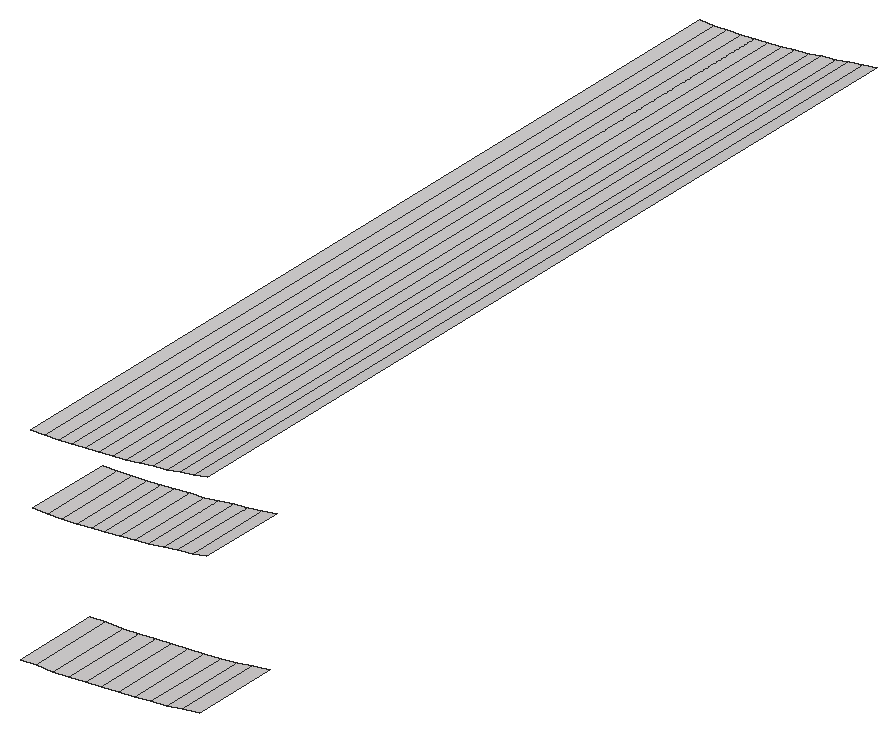
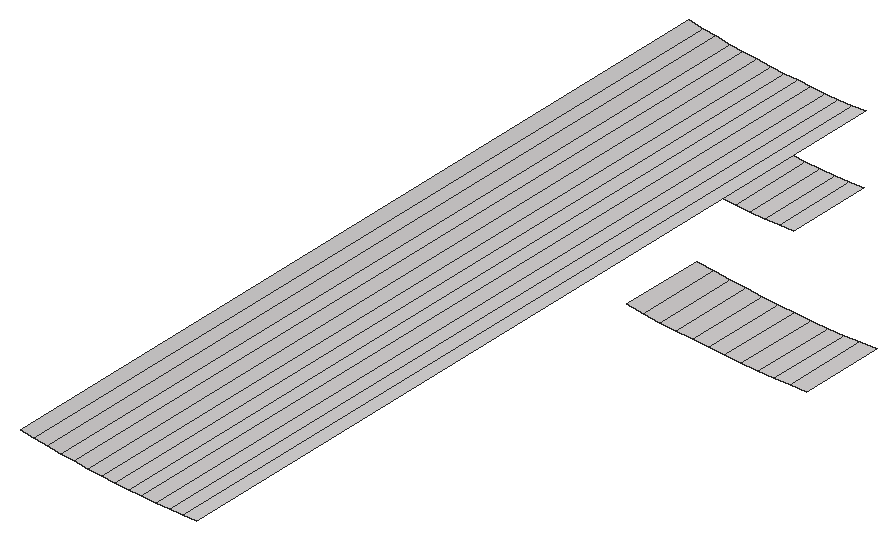
# SketchUp Ruby script. Lengths in inches.
U = 1.inch
M = Sketchup.active_model
def pt(a) = Geom::Point3d.new(a.map { |v| v * U })
def face(e, loops, mat)
  f = e.add_face(loops[0].map { |a| pt(a) })
  loops[1..].each { |l| e.add_face(l.map { |a| pt(a) }).erase! }
  f.material = f.back_material = mat if mat
  f
end
# faces: each face lists its corners as indices into pts; further lists are holes
def faces(e, pts, list, mat = nil) = list.each { |f| face(e, (f[0].is_a?(Array) ? f : [f]).map { |l| l.map { |i| pts[i] } }, mat) }
# xy, xz, yz: faces in a plane at the given z, y or x. An outline is a flat list of corners, or four numbers for a rectangle; further outlines are holes
def ring(l) = l.size == 4 ? [[l[0], l[1]], [l[2], l[1]], [l[2], l[3]], [l[0], l[3]]] : l.each_slice(2).to_a
def flat(e, list, mat, &to3) = list.each { |f| face(e, (f[0].is_a?(Array) ? f : [f]).map { |l| ring(l).map { |u, v| to3.(u, v) } }, mat) }
def xy(e, z, list, mat = nil) = flat(e, list, mat) { |x, y| [x, y, z] }
def xz(e, y, list, mat = nil) = flat(e, list, mat) { |x, z| [x, y, z] }
def yz(e, x, list, mat = nil) = flat(e, list, mat) { |y, z| [x, y, z] }
def lines(e, pts, list) = list.each { |a, b| e.add_line(pt(pts[a]), pt(pts[b])) }
# prism: a flat outline (further loops are holes) pulled along v
def prism(e, loops, v, mat = nil)
  f = face(e, loops, mat); d = Geom::Vector3d.new(v.map { |x| x * U })
  f.pushpull(f.normal.samedirection?(d) ? d.length : -d.length)
end
def box(e, o, s, mat = nil) = prism(e, [[o, [o[0] + s[0], o[1], o[2]], [o[0] + s[0], o[1] + s[1], o[2]], [o[0], o[1] + s[1], o[2]]]], [0, 0, s[2]], mat)
def at(x, y, z, deg = 0) = Geom::Transformation.translation(pt([x, y, z])) * Geom::Transformation.rotation(ORIGIN, Z_AXIS, deg.degrees)
def axes(o, x, y, z) = Geom::Transformation.new([*x, 0, *y, 0, *z, 0, *pt(o).to_a, 1])
def part(name) = M.definitions.add(name)
# library, detail: a bought-in or finely detailed component or shape, given as its bounding box
def library(name, o, s) = part(name).tap { |d| box(d.entities, o, s) }
def detail(e, o, s) = box(e.add_group.entities, o, s)
def put(e, d, t, mat = nil) = e.add_instance(d, t).tap { |i| i.material = mat if mat }
def group(e, t, mat = nil) = e.add_group.tap { |g| g.transformation = t; g.material = mat if mat }.entities
root = M.entities
M.materials.add("[Quartz Light Brown]").color = [215, 212, 212]
xy(root,150.01,[[450.47,143,450.71,144.25]],"[Quartz Light Brown]")
xy(root,152.01,[[450.42,143,450.63,144.25]],"[Quartz Light Brown]")
xy(root,153.01,[[450.39,143,450.59,155]],"[Quartz Light Brown]")
p = [[450.24,144.25,150],[450.24,143,150],[450.47,143,150.01],[450.47,144.25,150.01],[450.71,144.25,150.01],[450.71,143,150.01],
  [450.94,143,150.02],[450.94,144.25,150.02],[451.18,143,150.04],[451.18,144.25,150.04],[451.41,143,150.06],[451.41,144.25,150.06],
  [451.65,143,150.08],[451.65,144.25,150.08],[451.88,143,150.1],[451.88,144.25,150.1],[452.12,143,150.125],[452.12,144.25,150.125],
  [452.35,143,150.15],[452.35,144.25,150.15],[452.58,143,150.1875],[452.58,144.25,150.1875],[452.82,143,150.22],[452.82,144.25,150.22],
  [450.84,143,152.02],[450.63,143,152.01],[450.63,144.25,152.01],[450.84,144.25,152.02],[451.05,143,152.03],[451.05,144.25,152.03],
  [451.26,143,152.05],[451.26,144.25,152.05],[451.46,143,152.07],[451.46,144.25,152.07],[451.67,143,152.09],[451.67,144.25,152.09],
  [451.88,143,152.11],[451.88,144.25,152.11],[452.09,143,152.14],[452.09,144.25,152.14],[452.3,143,152.17],[452.3,144.25,152.17],
  [452.5,143,152.2],[452.5,144.25,152.2],[452.71,143,152.23],[452.71,144.25,152.23],[452.92,143,152.27],[452.92,144.25,152.27],
  [450.59,143,153.01],[450.79,143,153.02],[450.79,155,153.02],[450.59,155,153.01],[450.98,143,153.03],[450.98,155,153.03],
  [451.18,143,153.05],[451.18,155,153.05],[451.37,143,153.0625],[451.37,155,153.0625],[451.57,143,153.08],[451.57,155,153.08],
  [451.76,143,153.1],[451.76,155,153.1],[451.96,143,153.13],[451.96,155,153.13],[452.15,143,153.16],[452.15,155,153.16],
  [452.35,143,153.18],[452.35,155,153.18],[452.54,143,153.22],[452.54,155,153.22],[452.73,143,153.25],[452.73,155,153.25],
  [452.93,143,153.29],[452.93,155,153.29]]
faces(root,p,[[0,1,2,3],[4,5,6,7],[7,6,8,9],[9,8,10,11],[11,10,12,13],[13,12,14,15],[15,14,16,17],[17,16,18,19],
  [19,18,20,21],[21,20,22,23],[24,25,26,27],[28,24,27,29],[30,28,29,31],[32,30,31,33],[34,32,33,35],[36,34,35,37],
  [38,36,37,39],[40,38,39,41],[42,40,41,43],[44,42,43,45],[46,44,45,47],[48,49,50,51],[49,52,53,50],[52,54,55,53],
  [54,56,57,55],[56,58,59,57],[58,60,61,59],[60,62,63,61],[62,64,65,63],[64,66,67,65],[66,68,69,67],[68,70,71,69],
  [70,72,73,71]],"[Quartz Light Brown]")
